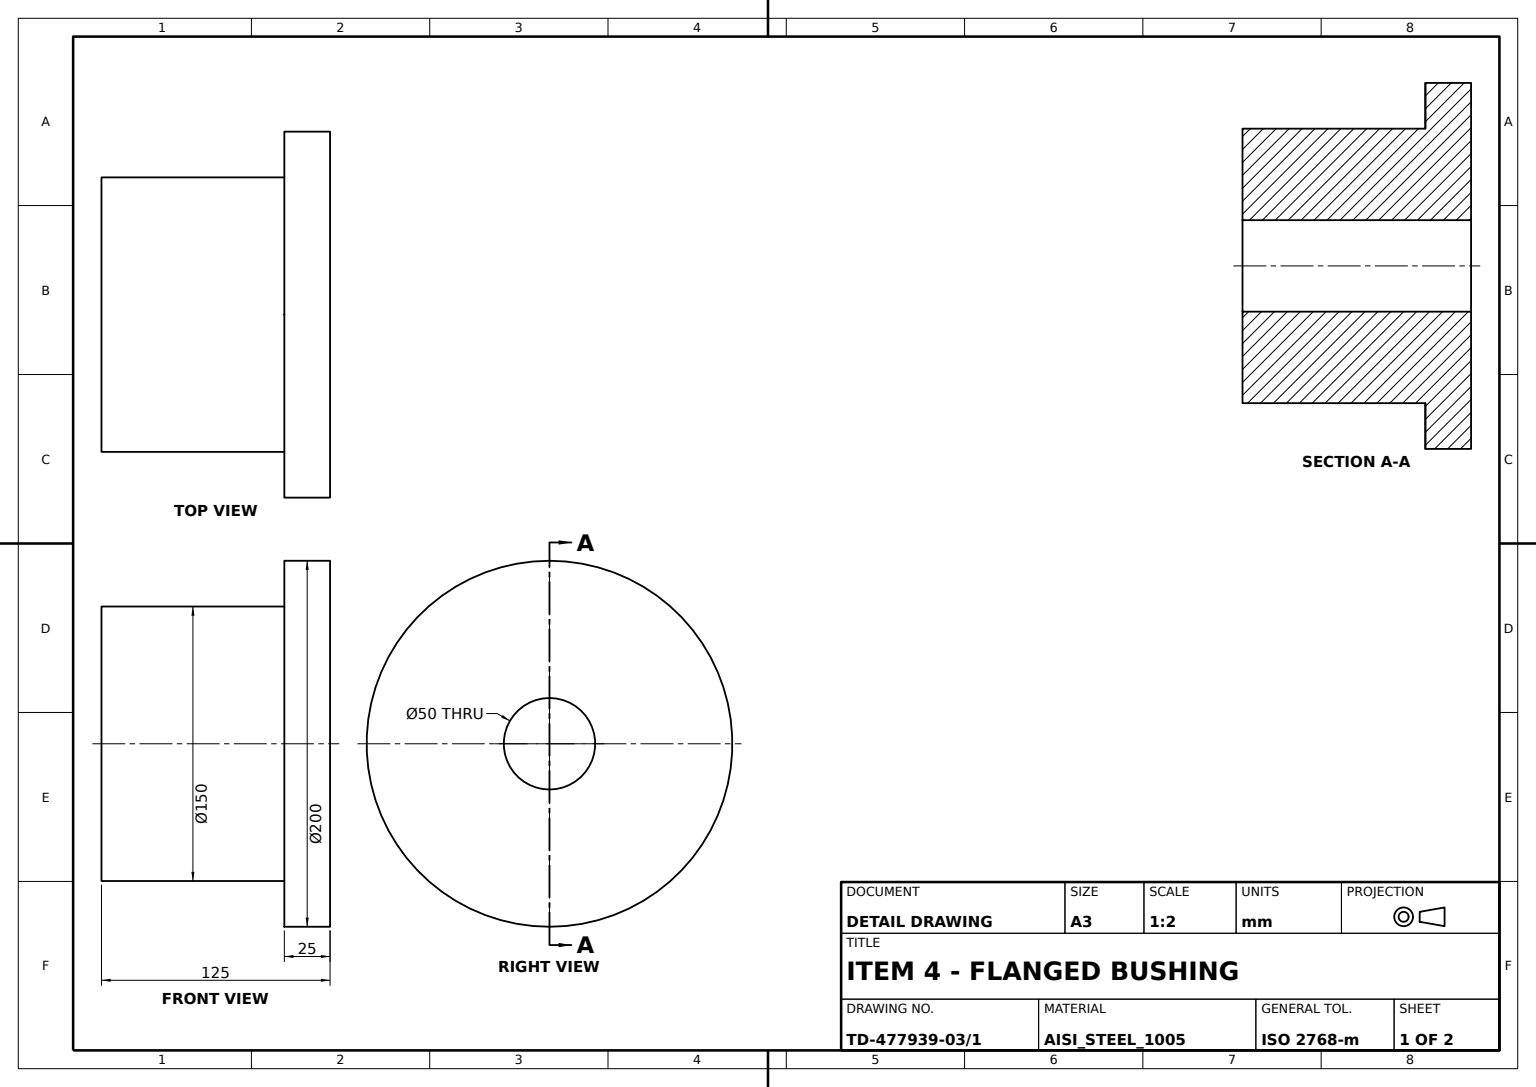
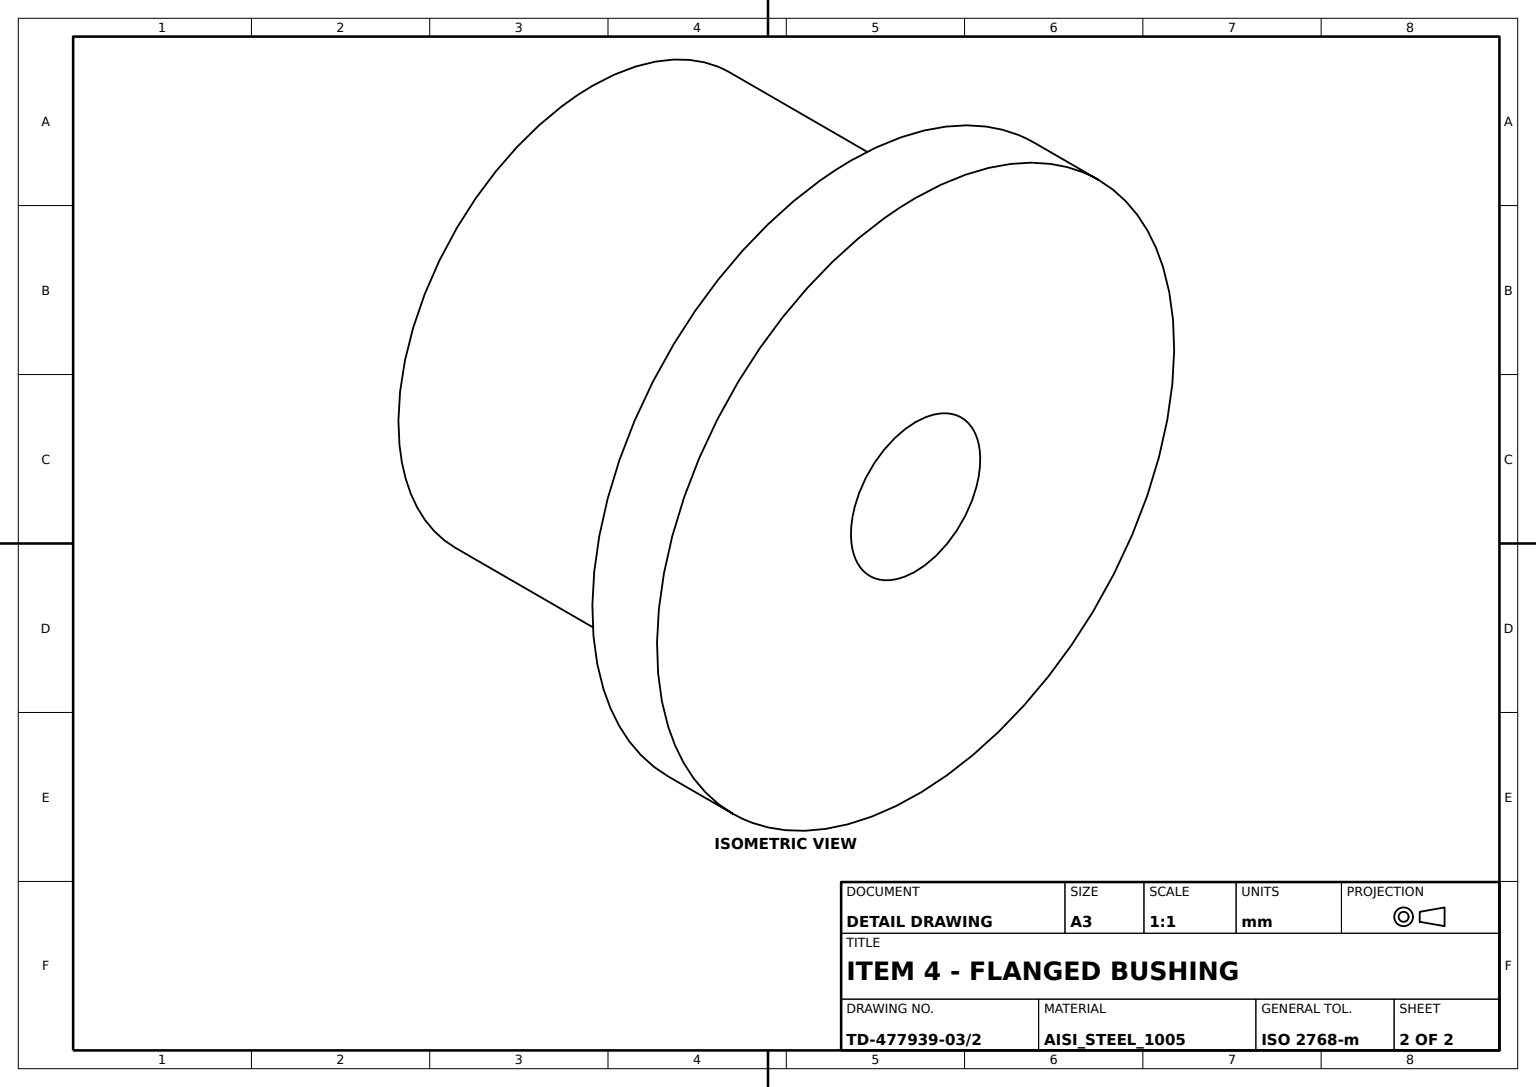
ISO-10303-21;
HEADER;
FILE_DESCRIPTION((''),'2;1');
FILE_NAME('','',(''),(''),'','','');
FILE_SCHEMA(('AUTOMOTIVE_DESIGN'));
ENDSEC;
DATA;
#1=APPLICATION_CONTEXT('');
#2=PRODUCT_CONTEXT('',#1,'mechanical');
#3=PRODUCT('','','',(#2));
#4=PRODUCT_DEFINITION_FORMATION('','',#3);
#5=PRODUCT_DEFINITION_CONTEXT('',#1,'design');
#6=PRODUCT_DEFINITION('','',#4,#5);
#7=PRODUCT_DEFINITION_SHAPE('','',#6);
#8=(LENGTH_UNIT()NAMED_UNIT(*)SI_UNIT(.MILLI.,.METRE.));
#9=(NAMED_UNIT(*)PLANE_ANGLE_UNIT()SI_UNIT($,.RADIAN.));
#10=(NAMED_UNIT(*)SI_UNIT($,.STERADIAN.)SOLID_ANGLE_UNIT());
#11=UNCERTAINTY_MEASURE_WITH_UNIT(LENGTH_MEASURE(0.005),#8,'distance_accuracy_value','');
#12=(GEOMETRIC_REPRESENTATION_CONTEXT(3)GLOBAL_UNCERTAINTY_ASSIGNED_CONTEXT((#11))GLOBAL_UNIT_ASSIGNED_CONTEXT((#8,#9,#10))REPRESENTATION_CONTEXT('',''));
#13=CARTESIAN_POINT('',(-75.,0.,0.));
#14=VERTEX_POINT('',#13);
#15=CARTESIAN_POINT('',(0.,0.,0.));
#16=DIRECTION('',(0.,0.,-1.));
#17=DIRECTION('',(-1.,0.,0.));
#18=AXIS2_PLACEMENT_3D('',#15,#16,#17);
#19=CIRCLE('',#18,75.);
#20=EDGE_CURVE('',#14,#14,#19,.T.);
#21=ORIENTED_EDGE('',*,*,#20,.T.);
#22=EDGE_LOOP('',(#21));
#23=FACE_BOUND('',#22,.T.);
#24=CARTESIAN_POINT('',(-25.,0.,0.));
#25=VERTEX_POINT('',#24);
#26=CIRCLE('',#18,25.);
#27=EDGE_CURVE('',#25,#25,#26,.T.);
#28=ORIENTED_EDGE('',*,*,#27,.F.);
#29=EDGE_LOOP('',(#28));
#30=FACE_BOUND('',#29,.T.);
#31=AXIS2_PLACEMENT_3D('',#24,#16,#17);
#32=PLANE('',#31);
#33=ADVANCED_FACE('',(#23,#30),#32,.T.);
#34=CARTESIAN_POINT('',(-100.,0.,100.));
#35=VERTEX_POINT('',#34);
#36=CARTESIAN_POINT('',(0.,0.,100.));
#37=AXIS2_PLACEMENT_3D('',#36,#16,#17);
#38=CIRCLE('',#37,100.);
#39=EDGE_CURVE('',#35,#35,#38,.T.);
#40=ORIENTED_EDGE('',*,*,#39,.F.);
#41=EDGE_LOOP('',(#40));
#42=FACE_BOUND('',#41,.T.);
#43=CARTESIAN_POINT('',(-100.,0.,125.));
#44=VERTEX_POINT('',#43);
#45=CARTESIAN_POINT('',(0.,0.,125.));
#46=AXIS2_PLACEMENT_3D('',#45,#16,#17);
#47=CIRCLE('',#46,100.);
#48=EDGE_CURVE('',#44,#44,#47,.T.);
#49=ORIENTED_EDGE('',*,*,#48,.T.);
#50=EDGE_LOOP('',(#49));
#51=FACE_BOUND('',#50,.T.);
#52=CYLINDRICAL_SURFACE('',#18,100.);
#53=ADVANCED_FACE('',(#42,#51),#52,.T.);
#54=ORIENTED_EDGE('',*,*,#27,.T.);
#55=EDGE_LOOP('',(#54));
#56=FACE_BOUND('',#55,.T.);
#57=CARTESIAN_POINT('',(-25.,0.,125.));
#58=VERTEX_POINT('',#57);
#59=CIRCLE('',#46,25.);
#60=EDGE_CURVE('',#58,#58,#59,.T.);
#61=ORIENTED_EDGE('',*,*,#60,.F.);
#62=EDGE_LOOP('',(#61));
#63=FACE_BOUND('',#62,.T.);
#64=CYLINDRICAL_SURFACE('',#18,25.);
#65=ADVANCED_FACE('',(#56,#63),#64,.F.);
#66=ORIENTED_EDGE('',*,*,#60,.T.);
#67=EDGE_LOOP('',(#66));
#68=FACE_BOUND('',#67,.T.);
#69=ORIENTED_EDGE('',*,*,#48,.F.);
#70=EDGE_LOOP('',(#69));
#71=FACE_BOUND('',#70,.T.);
#72=DIRECTION('',(0.,0.,1.));
#73=DIRECTION('',(1.,0.,0.));
#74=AXIS2_PLACEMENT_3D('',#43,#72,#73);
#75=PLANE('',#74);
#76=ADVANCED_FACE('',(#68,#71),#75,.T.);
#77=CARTESIAN_POINT('',(-75.,0.,100.));
#78=VERTEX_POINT('',#77);
#79=CIRCLE('',#37,75.);
#80=EDGE_CURVE('',#78,#78,#79,.T.);
#81=ORIENTED_EDGE('',*,*,#80,.F.);
#82=EDGE_LOOP('',(#81));
#83=FACE_BOUND('',#82,.T.);
#84=ORIENTED_EDGE('',*,*,#39,.T.);
#85=EDGE_LOOP('',(#84));
#86=FACE_BOUND('',#85,.T.);
#87=AXIS2_PLACEMENT_3D('',#77,#16,#17);
#88=PLANE('',#87);
#89=ADVANCED_FACE('',(#83,#86),#88,.T.);
#90=ORIENTED_EDGE('',*,*,#20,.F.);
#91=EDGE_LOOP('',(#90));
#92=FACE_BOUND('',#91,.T.);
#93=ORIENTED_EDGE('',*,*,#80,.T.);
#94=EDGE_LOOP('',(#93));
#95=FACE_BOUND('',#94,.T.);
#96=CYLINDRICAL_SURFACE('',#18,75.);
#97=ADVANCED_FACE('',(#92,#95),#96,.T.);
#98=CLOSED_SHELL('',(#33,#53,#65,#76,#89,#97));
#99=MANIFOLD_SOLID_BREP('',#98);
#100=ADVANCED_BREP_SHAPE_REPRESENTATION('',(#99),#12);
#101=SHAPE_DEFINITION_REPRESENTATION(#7,#100);
ENDSEC;
END-ISO-10303-21;
